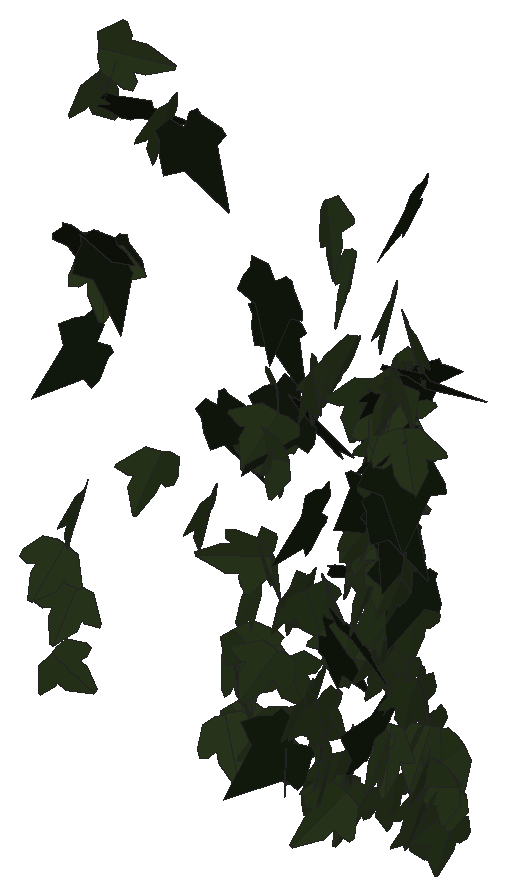
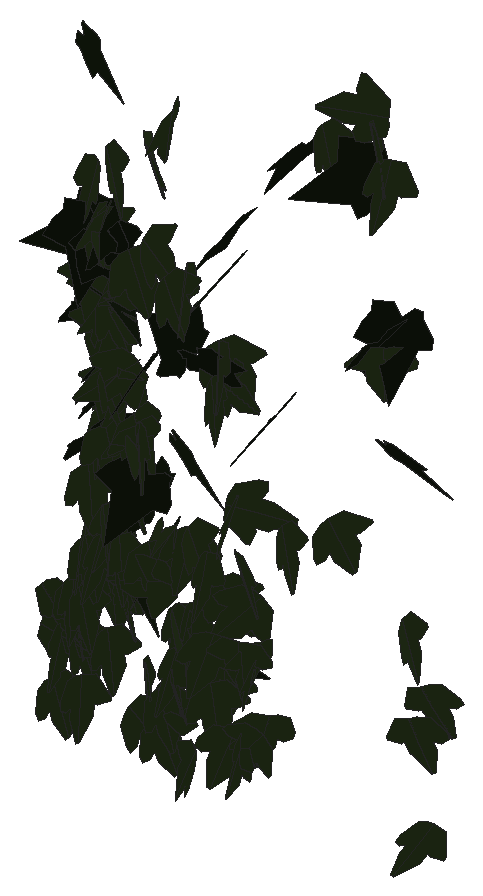
# SketchUp Ruby script. Lengths in inches.
U = 1.inch
M = Sketchup.active_model
def pt(a) = Geom::Point3d.new(a.map { |v| v * U })
def face(e, loops, mat)
  f = e.add_face(loops[0].map { |a| pt(a) })
  loops[1..].each { |l| e.add_face(l.map { |a| pt(a) }).erase! }
  f.material = f.back_material = mat if mat
  f
end
# faces: each face lists its corners as indices into pts; further lists are holes
def faces(e, pts, list, mat = nil) = list.each { |f| face(e, (f[0].is_a?(Array) ? f : [f]).map { |l| l.map { |i| pts[i] } }, mat) }
# xy, xz, yz: faces in a plane at the given z, y or x. An outline is a flat list of corners, or four numbers for a rectangle; further outlines are holes
def ring(l) = l.size == 4 ? [[l[0], l[1]], [l[2], l[1]], [l[2], l[3]], [l[0], l[3]]] : l.each_slice(2).to_a
def flat(e, list, mat, &to3) = list.each { |f| face(e, (f[0].is_a?(Array) ? f : [f]).map { |l| ring(l).map { |u, v| to3.(u, v) } }, mat) }
def xy(e, z, list, mat = nil) = flat(e, list, mat) { |x, y| [x, y, z] }
def xz(e, y, list, mat = nil) = flat(e, list, mat) { |x, z| [x, y, z] }
def yz(e, x, list, mat = nil) = flat(e, list, mat) { |y, z| [x, y, z] }
def lines(e, pts, list) = list.each { |a, b| e.add_line(pt(pts[a]), pt(pts[b])) }
# prism: a flat outline (further loops are holes) pulled along v
def prism(e, loops, v, mat = nil)
  f = face(e, loops, mat); d = Geom::Vector3d.new(v.map { |x| x * U })
  f.pushpull(f.normal.samedirection?(d) ? d.length : -d.length)
end
def box(e, o, s, mat = nil) = prism(e, [[o, [o[0] + s[0], o[1], o[2]], [o[0] + s[0], o[1] + s[1], o[2]], [o[0], o[1] + s[1], o[2]]]], [0, 0, s[2]], mat)
def at(x, y, z, deg = 0) = Geom::Transformation.translation(pt([x, y, z])) * Geom::Transformation.rotation(ORIGIN, Z_AXIS, deg.degrees)
def axes(o, x, y, z) = Geom::Transformation.new([*x, 0, *y, 0, *z, 0, *pt(o).to_a, 1])
def part(name) = M.definitions.add(name)
# library, detail: a bought-in or finely detailed component or shape, given as its bounding box
def library(name, o, s) = part(name).tap { |d| box(d.entities, o, s) }
def detail(e, o, s) = box(e.add_group.entities, o, s)
def put(e, d, t, mat = nil) = e.add_instance(d, t).tap { |i| i.material = mat if mat }
def group(e, t, mat = nil) = e.add_group.tap { |g| g.transformation = t; g.material = mat if mat }.entities
root = M.entities
M.materials.add("efeu1").color = [18, 25, 13]
M.materials.add("efeu2").color = [43, 57, 29]
c1 = part("ivyleaf_10")
p = [[0,0.5,-0.03],[-0.0625,2.02,-0.43],[-0.19,2.01,-0.46],[-0.54,1.05,-0.29],[-0.52,0.625,-0.18],[-0.83,0.76,-0.28],
  [-1.16,0.64,-0.33],[-1.15,0.33,-0.24],[-0.77,-0.39,0.02],[-0.3,-0.51,0.16],[0.04,-0.48,0.23],[-0.02,2.01,-0.4375],
  [-0.06,2.01,-0.43],[0.04,-0.49,0.23],[0.67,-0.49,0.14],[1.38,0.36,-0.2],[1.375,0.51,-0.24],[0.81,0.65,-0.19],
  [0.62,0.59,-0.15],[0.6,1.09,-0.28],[0.5,1.23,-0.31]]
faces(c1.entities,p,[[0,1,2,3,4,5,6,7,8,9,10],[11,12,0,13,14,15,16,17,18,19,20]],"efeu2")
c2 = part("ivyleaf_9")
p = [[1.54,2.16,1.25],[1.36,2.04,1.19],[-0.21,0.99,0.68],[-0.71,1.11,0.82],[-0.85,0.86,0.67],[-0.8,0.17,0.21],
  [-0.9,-0.01,0.1],[-0.67,-0.16,-0.02],[-0.08,-0.08,-0.05],[-0.03,-0.6,-0.4],[0.65,-0.88,-0.66],[0.83,-0.6,-0.49],
  [1.29,-0.42,-0.43],[1.8125,-0.07,-0.26],[1.21,0.44,0.15]]
faces(c2.entities,p,[[0,1,2,3,4,5,6,7,8,9,10,11,12,13,14]],"efeu1")
put(root,c1,axes([490.88,137.52,183.97],[-0.22065,-0.50459,-0.42857],[0.37535,0.27677,-0.51911],[0.54534,-0.39466,0.18389]))
put(root,c1,axes([491.52,136.6,187.67],[0.66402,0.10501,-0.25821],[-0.25401,-0.04675,-0.67224],[-0.11479,0.71092,-0.00607]))
put(root,c1,axes([491.93,136.6875,186.56],[0.67043,0.1776,-0.19159],[-0.19974,0.00838,-0.6912],[-0.16837,0.69722,0.05711]))
put(root,c1,axes([492.13,136.75,189.48],[0.21742,-0.70934,0.01301],[0.00528,-0.01199,-0.74191],[0.70944,0.21747,0.00153]))
put(root,c2,axes([493.03,136.25,194.59],[-0.76544,0.03807,-0.01605],[0.01216,-0.07694,-0.76259],[-0.03948,-0.76173,0.07623]))
put(root,c2,axes([493.35,135.53,198.16],[0.56258,0.38922,-0.38732],[-0.33855,-0.19072,-0.68339],[-0.43232,0.65585,0.03114]))
put(root,c1,axes([493.55,135.79,202.7],[-0.17337,-0.70311,-0.34039],[0.13336,0.31691,-0.72254],[0.7697,-0.21328,0.04852]))
put(root,c1,axes([493.46,136.07,197.24],[0.58317,0.51667,0.01827],[0.01457,0.0111,-0.77912],[-0.51679,0.58335,-0.00135]))
put(root,c2,axes([493.62,136.13,197.66],[0.06713,-0.76254,-0.11629],[-0.01109,0.11576,-0.76549],[0.77128,0.06803,-0.00089]))
put(root,c1,axes([494.08,135.68,203.65],[0.43656,-0.61324,-0.29097],[-0.13056,0.26363,-0.75151],[0.6661,0.45359,0.0434]))
put(root,c1,axes([494.82,136.56,191.58],[-0.32228,-0.59092,0.32145],[-0.01865,-0.34845,-0.65925],[0.67244,-0.29287,0.13577]))
put(root,c2,axes([494.3,135.57,202.36],[0.71441,0.01714,0.37317],[0.35644,0.20969,-0.69203],[-0.11177,0.77824,0.17824]))
put(root,c1,axes([494.43,135.29,204.06],[0.01324,-0.05693,0.81801],[0.707,0.41521,0.01746],[-0.41537,0.70492,0.05578]))
put(root,c1,axes([496,135.4,202.79],[0.09118,-0.79941,-0.00383],[-0.00086,0.00376,-0.80459],[0.79942,0.09118,-0.00043]))
put(root,c1,axes([496.36,136.72,190.84],[0.15284,-0.72412,-0.07115],[-0.00735,0.07116,-0.74003],[0.72757,0.15283,0.00746]))
put(root,c2,axes([496.64,135.53,202.42],[0.26973,-0.67391,-0.34362],[-0.0004,0.36469,-0.71553],[0.75646,0.24048,0.12215]))
put(root,c1,axes([497.03,137.25,184.6],[-0.54413,-0.05293,-0.45602],[0.45053,-0.19739,-0.51468],[-0.08817,-0.68196,0.18437]))
put(root,c1,axes([497.51,137.1875,184.09],[0.08162,-0.39829,-0.58429],[-0.04318,0.58426,-0.40431],[0.70581,0.0818,0.04283]))
put(root,c1,axes([497.27,136.4,184.68],[0.49721,0.52834,0.15021],[0.09579,0.11611,-0.72544],[-0.54087,0.50626,0.00961]))
put(root,c2,axes([497.18,136.22,194.14],[0.42939,-0.56864,-0.2736],[-0.07985,0.27931,-0.70583],[0.62596,0.4257,0.09764]))
put(root,c1,axes([497.63,136.41,186.78],[0.07931,0.70154,0.16436],[-0.01981,0.16742,-0.70501],[-0.72026,0.07264,0.03749]))
put(root,c1,axes([497.67,136.47,186.39],[-0.31882,0.64842,-0.01098],[0.00452,-0.01001,-0.72257],[-0.6485,-0.31886,0.00036]))
put(root,c1,axes([497.73,136.96,187.05],[0.6778,0.2556,0.04802],[0.04246,0.02348,-0.72435],[-0.25658,0.67909,0.00697]))
put(root,c1,axes([497.92,137.26,184.27],[-0.69218,-0.07129,-0.16335],[0.16205,0.02101,-0.69583],[0.07421,-0.71088,-0.00419]))
put(root,c1,axes([498.26,136.25,189.2],[0.49711,-0.47244,-0.27677],[-0.20397,0.18713,-0.68578],[0.50813,0.53731,-0.00452]))
put(root,c1,axes([498.73,135.6875,190.58],[0.09736,0.11008,-0.76258],[-0.76176,-0.10161,-0.11192],[-0.11564,0.76202,0.09524]))
put(root,c1,axes([498.18,135.98,187.84],[-0.56787,-0.13918,-0.48937],[0.48757,0.06068,-0.58303],[0.14537,-0.74718,0.04381]))
put(root,c1,axes([498.69,136.99,185.29],[-0.40361,-0.58965,0.08348],[-0.01375,-0.09159,-0.71343],[0.59537,-0.40185,0.04011]))
put(root,c1,axes([498.8125,136.02,190.66],[-0.39142,0.62615,0.11501],[-0.04082,0.11004,-0.73806],[-0.63532,-0.39285,-0.02343]))
put(root,c1,axes([498.82,136.96,186.76],[-0.41206,-0.53674,-0.26792],[0.2001,0.18344,-0.67526],[0.56554,-0.45598,0.04372]))
put(root,c1,axes([499.06,136.13,195.3],[0.46614,-0.40228,-0.47354],[-0.11904,0.5232,-0.56164],[0.60983,0.40962,0.25232]))
put(root,c1,axes([499.02,136.03,185.29],[-0.22818,-0.67276,-0.14966],[0.05354,0.13987,-0.71039],[0.68713,-0.23431,0.00565]))
put(root,c1,axes([499.29,135.68,187.75],[-0.51297,-0.34234,0.40403],[-0.24419,-0.34622,-0.60339],[0.4699,-0.55363,0.12751]))
put(root,c1,axes([499.27,137.25,183.2],[0.01441,0.1723,0.69331],[-0.41442,0.56687,-0.13226],[-0.58192,-0.39944,0.11136]))
put(root,c1,axes([499.0625,136.77,189.09],[0.07029,-0.64335,-0.36683],[0.07781,0.37286,-0.63901],[0.73648,0.02201,0.10252]))
put(root,c1,axes([499.52,135.44,194.89],[-0.58996,-0.36304,0.39935],[-0.26164,-0.32507,-0.68206],[0.47204,-0.63393,0.12106]))
put(root,c1,axes([499.77,135.28,194],[0.20492,-0.06423,-0.77113],[-0.70716,0.30834,-0.2136],[0.31417,0.73591,0.02219]))
put(root,c1,axes([499.43,135.98,194],[0.17189,-0.74457,0.00739],[0.12915,0.02234,-0.75287],[0.73332,0.17059,0.13086]))
put(root,c2,axes([499.72,136.18,195.07],[-0.73692,-0.22496,-0.02987],[0.02866,0.00844,-0.77049],[0.22512,-0.73748,0.00029]))
put(root,c1,axes([499.59,135.8,185.02],[0.43428,-0.41529,-0.4035],[-0.11459,0.43276,-0.56874],[0.56758,0.40513,0.19391]))
put(root,c2,axes([499.14,136.01,197.66],[0.34845,-0.69807,-0.06702],[0.0147,0.08209,-0.77862],[0.70113,0.34521,0.04963]))
put(root,c1,axes([499.61,136.63,189.66],[0.12678,-0.72667,0.12442],[-0.00085,-0.12639,-0.73731],[0.73724,0.12482,-0.02224]))
put(root,c2,axes([499.28,135.84,198.71],[0.05549,-0.75516,0.22128],[0.0123,-0.22097,-0.75719],[0.78682,0.05671,-0.00377]))
put(root,c2,axes([499.83,135.79,185.41],[-0.56518,-0.43403,0.27698],[-0.19407,-0.20137,-0.71155],[0.4769,-0.59631,0.03868]))
put(root,c1,axes([499.91,136.46,189.4375],[-0.33863,-0.62476,-0.21716],[0.14805,0.16617,-0.70895],[0.64464,-0.36635,0.04875]))
put(root,c1,axes([500,136.83,187.04],[0.27996,-0.67818,0.01963],[-0.00097,-0.02164,-0.73363],[0.67846,0.27981,-0.00914]))
put(root,c1,axes([500.03,136.97,185.83],[0.0215,-0.56387,-0.46352],[0.07673,0.46289,-0.55955],[0.72589,-0.03222,0.07288]))
put(root,c1,axes([499.88,137.05,185.14],[0.45447,-0.46224,0.32748],[0.24473,-0.21843,-0.64796],[0.5109,0.51582,0.01908]))
put(root,c2,axes([500.4,136.26,192.15],[-0.65391,0.36445,-0.12591],[0.10341,-0.07305,-0.7485],[-0.37146,-0.66191,0.01327]))
put(root,c1,axes([500.22,135.87,186.71],[0.06133,-0.68795,-0.34016],[0.00205,0.34139,-0.69007],[0.76745,0.05407,0.02903]))
put(root,c1,axes([500.32,137.1875,183.74],[-0.28505,-0.6104,0.24274],[-0.0069,-0.26182,-0.66646],[0.65686,-0.26764,0.09835]))
put(root,c1,axes([500.38,137.03,184.54],[-0.15425,-0.69934,0.08715],[-0.01981,-0.08488,-0.71615],[0.70447,-0.15552,-0.00106]))
put(root,c1,axes([500.55,136.02,186.64],[-0.07512,-0.70973,-0.23758],[0.04151,0.23446,-0.71352],[0.74729,-0.08436,0.01575]))
put(root,c1,axes([500.9,136.65,188.76],[-0.47906,0.36937,-0.43856],[-0.35779,0.25401,0.60476],[0.44806,0.59775,0.01401]))
put(root,c1,axes([500.9,136.06,196.66],[0.00767,-0.75781,0.18894],[0.03003,-0.18852,-0.75736],[0.78043,0.0147,0.02728]))
put(root,c1,axes([500.88,135.3,196.72],[0.27923,-0.6487,-0.33393],[0.06226,0.37743,-0.68115],[0.72694,0.21686,0.18661]))
put(root,c1,axes([500.95,136.95,185.19],[0.38904,-0.59205,-0.15393],[0.01234,0.18998,-0.69951],[0.61161,0.37276,0.11203]))
put(root,c2,axes([500.39,136.03,194.94],[0.23335,-0.40053,0.61952],[0.46081,-0.42829,-0.45045],[0.5761,0.50481,0.10937]))
put(root,c1,axes([501.08,136.66,188.66],[-0.44107,-0.58454,0.14421],[0.01086,-0.18646,-0.7226],[0.60197,-0.42494,0.1187]))
put(root,c1,axes([501.15,136.03,184.02],[0.26568,0.38314,-0.61383],[-0.36451,-0.494,-0.46611],[-0.62507,0.45092,0.01091]))
put(root,c1,axes([501.16,135.62,185.32],[0.39113,-0.6209,-0.24164],[-0.07793,0.23565,-0.73164],[0.66169,0.39477,0.05667]))
put(root,c1,axes([501.25,137.01,183.79],[-0.09198,-0.59474,0.39006],[-0.04711,-0.38735,-0.60172],[0.70968,-0.1028,0.01061]))
put(root,c2,axes([501.03,135.88,188.89],[0.52008,-0.2853,-0.47806],[-0.36621,0.31744,-0.58783],[0.41933,0.63108,0.07956]))
put(root,c1,axes([500.7,136.71,188.03],[-0.14115,-0.01399,-0.72946],[0.72622,0.06866,-0.14184],[0.07007,-0.73981,0.00063]))
put(root,c1,axes([501.35,135.54,201.58],[-0.16144,0.76906,-0.17946],[0.01313,-0.18053,-0.78547],[-0.78961,-0.16023,0.02363]))
put(root,c2,axes([501.42,136.4375,190.89],[0.57378,0.49687,0.00466],[-0.0968,0.11876,-0.7434],[-0.48737,0.56137,0.15315]))
put(root,c1,axes([501.65,135.89,197.62],[0.15203,-0.66536,0.39424],[0.08102,-0.38587,-0.68248],[0.76913,0.17217,-0.00604]))
put(root,c1,axes([501.71,136.3,192],[0.49363,-0.49893,-0.30782],[-0.07619,0.3444,-0.6804],[0.58127,0.46884,0.17223]))
put(root,c1,axes([501.85,136.35,191.79],[0.20146,-0.68889,0.26418],[0.05663,-0.25861,-0.71754],[0.73563,0.20857,-0.01711]))
put(root,c1,axes([501.92,136.25,192.3],[0.15255,0.71243,-0.24275],[-0.19212,-0.20262,-0.7154],[-0.72772,0.20284,0.13798]))
put(root,c1,axes([502.05,136.7,188.54],[0.05425,-0.72495,-0.16649],[-0.00976,0.16623,-0.72697],[0.74376,0.05506,0.0026]))
put(root,c1,axes([501.89,136.31,192.02],[0.23622,0.71549,-0.13948],[-0.03748,-0.13451,-0.75345],[-0.728,0.23909,-0.00647]))
put(root,c1,axes([501.95,135.54,200.31],[0.57677,-0.51262,0.2237],[0.15234,-0.16521,-0.77135],[0.53816,0.59616,-0.0214]))
put(root,c1,axes([502.46,135.7,196.79],[-0.3354,-0.69105,0.19205],[-0.05228,-0.18789,-0.7674],[0.71534,-0.33775,0.03397]))
put(root,c1,axes([502.61,135.88,190.23],[0.55032,-0.39006,-0.3983],[-0.31469,0.24463,-0.67436],[0.46017,0.63376,0.01516]))
put(root,c2,axes([501.83,135.6,189.63],[0.40883,-0.53526,0.38014],[0.29625,-0.24923,-0.66954],[0.58587,0.49954,0.07329]))
put(root,c2,axes([502.21,136.16,193.21],[0.35175,-0.41941,-0.54577],[0.33227,-0.4333,0.54712],[-0.6028,-0.48357,-0.01689]))
put(root,c1,axes([502.36,135.89,191.15],[0.16998,-0.54115,0.49831],[0.23662,-0.44404,-0.56293],[0.69654,0.28291,0.06963]))
put(root,c2,axes([503.02,135.1875,186.96],[-0.38433,0.61801,0.33207],[-0.19153,0.27183,-0.72756],[-0.67492,-0.42906,0.01737]))
put(root,c1,axes([502.71,136.53,189.14],[0.25112,-0.6677,-0.2251],[-0.04921,0.22177,-0.71271],[0.7029,0.25407,0.03052]))
put(root,c1,axes([502.4,136.11,193.72],[-0.37825,-0.2227,-0.63961],[0.54706,0.33142,-0.43892],[0.39927,-0.66508,-0.00455]))
put(root,c1,axes([502.87,136.18,193.3],[0.13104,-0.75965,0.0594],[0.00202,-0.05993,-0.77082],[0.76196,0.1308,-0.00817]))
put(root,c1,axes([502.59,136.13,193.35],[0.653,0.3271,0.26082],[0.16926,0.23557,-0.71923],[-0.38258,0.66253,0.12697]))
put(root,c1,axes([502.93,135.97,195.48],[-0.08417,-0.76029,0.17337],[0.00263,-0.17465,-0.76463],[0.7798,-0.08148,0.02129]))
put(root,c1,axes([502.9375,136.1,185.1],[-0.11889,-0.71558,-0.0452],[0.00909,0.04431,-0.72539],[0.71695,-0.11923,0.0017]))
put(root,c1,axes([503,136.14,191.47],[-0.42977,-0.6068,0.16225],[0.03102,-0.21686,-0.72886],[0.62735,-0.40497,0.14719]))
put(root,c1,axes([503.02,135.53,186.6],[0.5874,-0.51934,-0.13296],[-0.09238,0.09624,-0.78399],[0.52807,0.59452,0.01076]))
put(root,c2,axes([503.51,135.35,195.62],[-0.23004,0.64026,0.29786],[-0.30108,0.19738,-0.67452],[-0.69511,-0.29738,0.19359]))
put(root,c1,axes([502.99,136.47,188.11],[0.0395,-0.63707,-0.38176],[0.1307,0.3823,-0.62444],[0.73111,-0.03392,0.13226]))
put(root,c1,axes([503.03,135.88,188.82],[-0.1284,-0.62417,-0.3879],[0.13673,0.36661,-0.63517],[0.72205,-0.18042,0.0513]))
put(root,c1,axes([503.11,135.79,196.06],[0.5648,0.5157,-0.19304],[-0.12733,-0.14672,-0.7645],[-0.53572,0.57856,-0.0218]))
put(root,c1,axes([502.98,135.83,186.65],[0.74692,-0.05179,0.1256],[0.12549,-0.00583,-0.74871],[0.05204,0.75738,0.00283]))
put(root,c2,axes([503.49,135.76,197.3],[-0.22859,0.58321,-0.48952],[-0.01791,-0.51508,-0.6053],[-0.76121,-0.16301,0.16124]))
put(root,c1,axes([503.27,136.85,186.59],[0.02882,-0.73569,-0.00337],[-0.00007,0.00337,-0.73625],[0.73569,0.02882,0.00006]))
put(root,c1,axes([503.28,135.59,199.64],[0.31106,-0.7327,-0.08513],[-0.02097,0.08356,-0.79589],[0.73733,0.31148,0.01328]))
put(root,c1,axes([503.28,136.89,183.88],[-0.15515,-0.68174,-0.17317],[0.03717,0.16914,-0.69917],[0.70241,-0.15954,-0.00125]))
put(root,c1,axes([503.13,135.94,195.33],[-0.01237,0.78489,-0.00492],[0.00632,-0.00482,-0.78496],[-0.78488,-0.01241,-0.00624]))
put(root,c1,axes([503.01,136.01,195.03],[0.66202,0.34794,0.23836],[0.15541,0.21117,-0.73986],[-0.39208,0.67119,0.10921]))
put(root,c1,axes([503.12,135.91,196.21],[0.35893,0.62564,0.32056],[0.01286,0.35402,-0.70535],[-0.70286,0.32597,0.1508]))
put(root,c1,axes([503.36,136.49,187.98],[-0.16427,-0.72316,0.04762],[0.00748,-0.05052,-0.74135],[0.72469,-0.16341,0.01845]))
put(root,c2,axes([503.1,136.25,192.82],[-0.07827,-0.6945,0.32015],[0.00805,-0.32255,-0.69775],[0.7647,-0.06769,0.04012]))
put(root,c1,axes([503.42,136.36,190.11],[-0.27573,-0.70069,-0.03012],[0.0058,0.03008,-0.75296],[0.70131,-0.27573,-0.00562]))
put(root,c1,axes([503.54,135.73,197.5],[-0.0517,-0.69287,0.38897],[0.02269,-0.39092,-0.69333],[0.79426,-0.03393,0.04512]))
put(root,c2,axes([503.1875,135.64,193.75],[0.32401,-0.62124,-0.31863],[-0.08437,0.31385,-0.69772],[0.69307,0.32864,0.06402]))
put(root,c1,axes([503.5625,135.65,191.53],[0.03489,-0.71905,-0.24535],[0.05126,0.24728,-0.71741],[0.75803,0.01638,0.05981]))
put(root,c2,axes([503.45,136.34,191.43],[-0.20782,-0.71014,0.17606],[-0.0452,-0.17021,-0.73991],[0.73024,-0.21264,0.0043]))
put(root,c1,axes([503.59,136.82,186.79],[0.0057,-0.70385,-0.21452],[0.0587,0.21428,-0.7015],[0.73347,-0.01168,0.05781]))
put(root,c1,axes([503.54,135.74,197.57],[0.23954,-0.63784,0.41313],[0.14451,-0.38703,-0.68134],[0.74608,0.27976,-0.00067]))
put(root,c1,axes([503.62,136.27,188.15],[0.21916,-0.61722,-0.35918],[0.04467,0.38683,-0.63748],[0.71273,0.16555,0.1504]))
put(root,c1,axes([503.71,136.53,186.62],[-0.41672,-0.55756,0.23996],[0.02565,-0.30698,-0.66874],[0.60646,-0.37013,0.19317]))
put(root,c1,axes([503.71,136.3,184.94],[0.02976,-0.74264,0.11593],[0.00019,-0.11601,-0.74323],[0.75164,0.02943,-0.0044]))
put(root,c1,axes([503.5625,135.73,197.76],[-0.17118,0.77991,-0.00669],[0.00562,-0.00562,-0.79846],[-0.77992,-0.17122,-0.00428]))
put(root,c2,axes([503.8,135.71,197.64],[0.32,0.72404,-0.0972],[-0.03164,-0.09228,-0.79155],[-0.72985,0.32145,-0.0083]))
put(root,c1,axes([503.9375,137.18,183.75],[-0.19718,-0.67574,0.13557],[-0.01886,-0.13567,-0.70365],[0.68895,-0.19711,0.01954]))
put(root,c1,axes([503.94,136.18,186.01],[0.27212,-0.65517,-0.26788],[-0.08041,0.25652,-0.70908],[0.70324,0.28285,0.02258]))
put(root,c1,axes([503.99,135.15,191.97],[0.11322,-0.55693,-0.58004],[-0.08954,0.57339,-0.56802],[0.79913,0.14316,0.01854]))
put(root,c1,axes([503.98,135.58,199.03],[-0.64051,0.47934,0.07627],[-0.06309,0.04299,-0.80001],[-0.48125,-0.6436,0.00337]))
put(root,c1,axes([504.47,136.61,185.2],[0.19637,0.02791,-0.7104],[-0.70014,0.13556,-0.18821],[0.12345,0.72446,0.06258]))
put(root,c2,axes([504.22,135.51,203.04],[-0.54967,0.38337,-0.29496],[0.23845,-0.17822,-0.66261],[-0.4565,-0.55471,0.00904]))
put(root,c2,axes([503.86,135.59,195.08],[-0.2494,-0.71427,-0.17879],[0.07017,0.16485,-0.75647],[0.73295,-0.25883,0.01159]))
put(root,c2,axes([503.44,135.76,197.51],[0.67504,-0.14654,0.39692],[0.42138,0.16539,-0.65558],[0.03819,0.76542,0.21765]))
put(root,c1,axes([504.1,136.68,185.09],[0.04495,-0.62259,-0.38285],[0.0713,0.38548,-0.61849],[0.7274,0.00069,0.08428]))
put(root,c1,axes([504.4,136.8,186.38],[0.51856,-0.09953,-0.48932],[-0.45486,0.19687,-0.52209],[0.206,0.68525,0.07893]))
put(root,c1,axes([504.58,136.24,185.61],[0.27723,-0.10146,-0.66559],[-0.64623,0.22708,-0.28704],[0.26858,0.65109,-0.00361]))
put(root,c1,axes([503.9375,135.34,195.89],[0.6876,0.34312,0.15094],[0.0728,0.17654,-0.74156],[-0.39571,0.62869,0.12586]))
